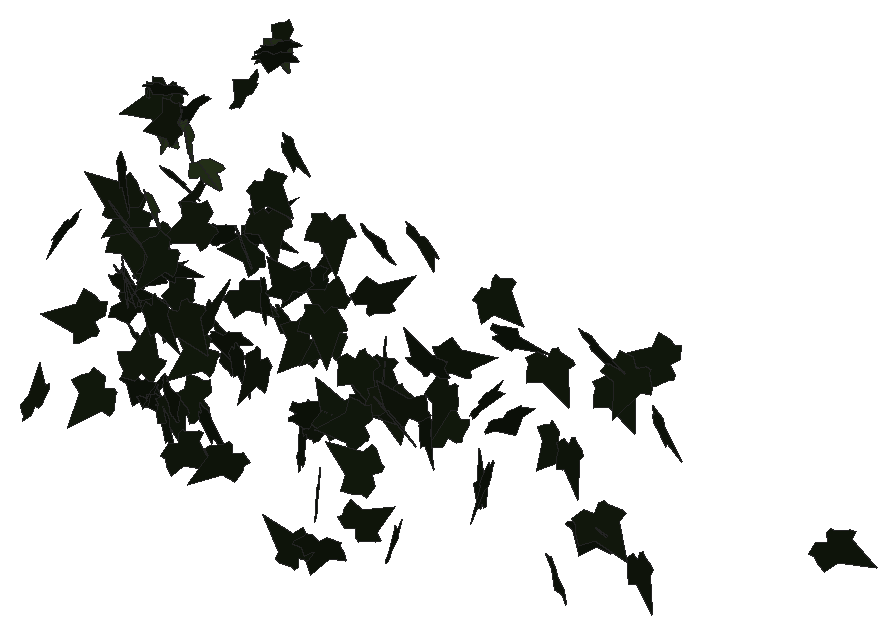
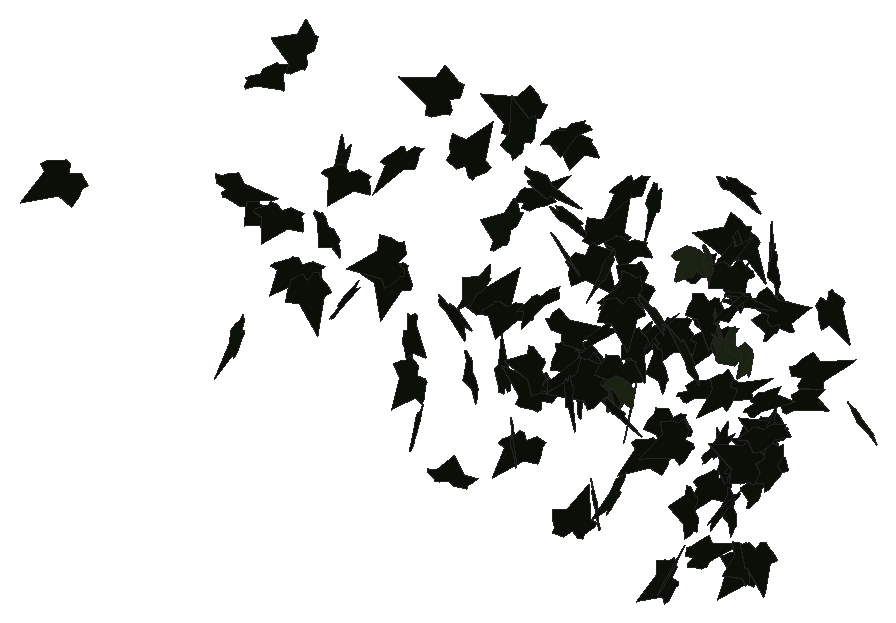
# SketchUp Ruby script. Lengths in inches.
U = 1.inch
M = Sketchup.active_model
def pt(a) = Geom::Point3d.new(a.map { |v| v * U })
def face(e, loops, mat)
  f = e.add_face(loops[0].map { |a| pt(a) })
  loops[1..].each { |l| e.add_face(l.map { |a| pt(a) }).erase! }
  f.material = f.back_material = mat if mat
  f
end
# faces: each face lists its corners as indices into pts; further lists are holes
def faces(e, pts, list, mat = nil) = list.each { |f| face(e, (f[0].is_a?(Array) ? f : [f]).map { |l| l.map { |i| pts[i] } }, mat) }
# xy, xz, yz: faces in a plane at the given z, y or x. An outline is a flat list of corners, or four numbers for a rectangle; further outlines are holes
def ring(l) = l.size == 4 ? [[l[0], l[1]], [l[2], l[1]], [l[2], l[3]], [l[0], l[3]]] : l.each_slice(2).to_a
def flat(e, list, mat, &to3) = list.each { |f| face(e, (f[0].is_a?(Array) ? f : [f]).map { |l| ring(l).map { |u, v| to3.(u, v) } }, mat) }
def xy(e, z, list, mat = nil) = flat(e, list, mat) { |x, y| [x, y, z] }
def xz(e, y, list, mat = nil) = flat(e, list, mat) { |x, z| [x, y, z] }
def yz(e, x, list, mat = nil) = flat(e, list, mat) { |y, z| [x, y, z] }
def lines(e, pts, list) = list.each { |a, b| e.add_line(pt(pts[a]), pt(pts[b])) }
# prism: a flat outline (further loops are holes) pulled along v
def prism(e, loops, v, mat = nil)
  f = face(e, loops, mat); d = Geom::Vector3d.new(v.map { |x| x * U })
  f.pushpull(f.normal.samedirection?(d) ? d.length : -d.length)
end
def box(e, o, s, mat = nil) = prism(e, [[o, [o[0] + s[0], o[1], o[2]], [o[0] + s[0], o[1] + s[1], o[2]], [o[0], o[1] + s[1], o[2]]]], [0, 0, s[2]], mat)
def at(x, y, z, deg = 0) = Geom::Transformation.translation(pt([x, y, z])) * Geom::Transformation.rotation(ORIGIN, Z_AXIS, deg.degrees)
def axes(o, x, y, z) = Geom::Transformation.new([*x, 0, *y, 0, *z, 0, *pt(o).to_a, 1])
def part(name) = M.definitions.add(name)
# library, detail: a bought-in or finely detailed component or shape, given as its bounding box
def library(name, o, s) = part(name).tap { |d| box(d.entities, o, s) }
def detail(e, o, s) = box(e.add_group.entities, o, s)
def put(e, d, t, mat = nil) = e.add_instance(d, t).tap { |i| i.material = mat if mat }
def group(e, t, mat = nil) = e.add_group.tap { |g| g.transformation = t; g.material = mat if mat }.entities
root = M.entities
M.materials.add("efeu1").color = [18, 25, 13]
M.materials.add("efeu2").color = [43, 57, 29]
c1 = part("ivyleaf_9")
p = [[1.54,2.16,1.25],[1.36,2.04,1.19],[-0.21,0.99,0.68],[-0.71,1.11,0.82],[-0.85,0.86,0.67],[-0.8,0.17,0.21],
  [-0.9,-0.01,0.1],[-0.67,-0.16,-0.02],[-0.08,-0.08,-0.05],[-0.03,-0.6,-0.4],[0.65,-0.88,-0.66],[0.83,-0.6,-0.49],
  [1.29,-0.42,-0.43],[1.8125,-0.07,-0.26],[1.21,0.44,0.15]]
faces(c1.entities,p,[[0,1,2,3,4,5,6,7,8,9,10,11,12,13,14]],"efeu1")
c2 = part("ivyleaf_10")
p = [[0,0.5,-0.03],[-0.0625,2.02,-0.43],[-0.19,2.01,-0.46],[-0.54,1.05,-0.29],[-0.52,0.625,-0.18],[-0.83,0.76,-0.28],
  [-1.16,0.64,-0.33],[-1.15,0.33,-0.24],[-0.77,-0.39,0.02],[-0.3,-0.51,0.16],[0.04,-0.48,0.23],[-0.02,2.01,-0.4375],
  [-0.06,2.01,-0.43],[0.04,-0.49,0.23],[0.67,-0.49,0.14],[1.38,0.36,-0.2],[1.375,0.51,-0.24],[0.81,0.65,-0.19],
  [0.62,0.59,-0.15],[0.6,1.09,-0.28],[0.5,1.23,-0.31]]
faces(c2.entities,p,[[0,1,2,3,4,5,6,7,8,9,10],[11,12,0,13,14,15,16,17,18,19,20]],"efeu2")
put(root,c1,axes([629.57,122.1,292.07],[-0.71361,-0.84052,0.81421],[-0.5253,-0.62208,-1.10259],[1.04568,-0.8861,0.00175]))
put(root,c1,axes([629.91,140.37,299.85],[-1.23005,0.22373,0.09712],[-0.09277,0.03263,-1.25014],[-0.22557,-1.23345,-0.01545]))
put(root,c1,axes([628.84,122,289.8],[-0.35154,-1.20696,-0.64325],[0.29676,0.58102,-1.25238],[1.33509,-0.44695,0.109]))
put(root,c1,axes([628.47,121.0625,286.31],[1.21635,-0.61794,0.36407],[0.32919,-0.15581,-1.36428],[0.63721,1.26007,0.00984]))
put(root,c1,axes([630.87,123.4375,301.76],[-1.0355,-0.05838,0.68681],[-0.66838,-0.21794,-1.02623],[0.16849,-1.2233,0.15005]))
put(root,c1,axes([629.83,125.12,302.06],[0.0302,-1.23454,0.00848],[0.00022,-0.00847,-1.23491],[1.23457,0.0302,0.00002]))
put(root,c2,axes([630.18,125.09,298.99],[-0.01245,0.99855,-0.72682],[-0.09137,-0.72561,-0.99533],[-1.23168,0.04374,0.08118]))
put(root,c2,axes([629.45,125.24,297.93],[0.68687,-0.12482,-1.01492],[1.01721,-0.04157,0.69353],[-0.10453,-1.22479,0.07989]))
put(root,c1,axes([630.79,120.64,277.54],[0.62969,0.60238,-0.88819],[-0.69997,-0.55008,-0.86932],[-0.8135,0.93958,0.06049]))
put(root,c1,axes([630.78,111.37,296.12],[-0.62437,0.95631,-0.70967],[0.367,-0.60778,-1.14189],[-1.1329,-0.72393,0.02121]))
put(root,c2,axes([630.31,138.29,300.37],[-1.17005,0.09928,-0.46292],[0.46073,-0.04536,-1.17424],[-0.10899,-1.25748,0.00581]))
put(root,c1,axes([630.16,124.96,294.55],[1.21698,-0.1043,-0.08314],[-0.07304,0.11741,-1.21644],[0.11161,1.21416,0.11049]))
put(root,c1,axes([630.16,121.86,286.3],[0.54823,1.03089,-0.57968],[0.25524,0.52075,1.16748],[1.15483,-0.60449,0.01715]))
put(root,c1,axes([631.6,122.72,303.88],[0.33423,1.02024,-0.62057],[-0.66252,-0.37772,-0.97781],[-0.99351,0.5951,0.44328]))
put(root,c1,axes([630.5625,118.77,285.53],[0.0714,0.52873,-1.29242],[0.13606,1.28531,0.53334],[1.38974,-0.153,0.01419]))
put(root,c1,axes([631.45,136.85,301.32],[0.5126,1.13395,-0.20258],[-0.2832,-0.09087,-1.22523],[-1.11655,0.54364,0.21776]))
put(root,c1,axes([632,105.65,282.48],[-1.0933,0.60329,-0.55811],[-0.49299,0.26175,1.24868],[0.65757,1.19928,0.00822]))
put(root,c2,axes([631.27,124.99,300.29],[0.83224,-0.89057,0.22858],[0.23725,-0.08987,-1.21393],[0.8883,0.85837,0.11006]))
put(root,c1,axes([631.59,120.84,276.31],[0.27096,0.53541,1.09573],[0.28579,1.06331,-0.59025],[-1.18558,0.37868,0.10814]))
put(root,c1,axes([630.96,119.13,287.47],[0.28732,-0.78886,0.90976],[0.31923,-0.85193,-0.83953],[1.16106,0.42945,0.0057]))
put(root,c1,axes([630.61,118.55,286.83],[0.47734,-0.33274,1.16148],[1.0531,-0.49756,-0.57534],[0.59222,1.15296,0.08691]))
put(root,c1,axes([632.98,116.08,296.46],[-0.20572,0.1631,1.47402],[-1.37992,0.52409,-0.25058],[-0.54327,-1.39298,0.07831]))
put(root,c1,axes([632.29,124.83,301.41],[0.09194,1.23358,-0.1325],[-0.00712,-0.13234,-1.237],[-1.24066,0.09217,-0.00272]))
put(root,c1,axes([631.58,120.79,276.125],[1.17324,0.42953,-0.0039],[-0.00984,0.01552,-1.24927],[-0.42943,1.17315,0.01795]))
put(root,c2,axes([631.95,120.25,294.83],[-0.98739,0.68872,-0.31477],[0.2713,-0.16117,-1.20365],[-0.70698,-1.02374,-0.02227]))
put(root,c1,axes([631.375,119.42,282.46],[0.68949,-0.85409,0.56382],[0.34676,-0.44466,-1.09764],[0.96287,0.77173,-0.00845]))
put(root,c1,axes([633.52,111.03,288.29],[-0.44671,-0.19552,1.39444],[-1.28089,-0.55116,-0.48761],[0.58481,-1.35655,-0.00286]))
put(root,c1,axes([633.49,120.41,291.02],[-0.5655,-0.94835,-0.6007],[-0.30568,-0.51711,1.10415],[-1.08017,0.64282,0.00202]))
put(root,c1,axes([633.6,128.8,277.14],[0.08869,-1.24031,0.50443],[0.08246,0.50964,1.23862],[-1.33643,-0.05086,0.1099]))
put(root,c1,axes([632.7,115.52,295.73],[0.84734,-0.83471,0.6193],[0.43527,-0.4406,-1.1894],[0.94383,0.95257,-0.00747]))
put(root,c1,axes([632.91,115.4375,300.49],[-0.2181,0.04436,-1.40532],[1.39566,-0.16546,-0.22182],[-0.17034,-1.41249,-0.01815]))
put(root,c1,axes([634.13,121.86,285.78],[-0.4084,-1.08907,0.62257],[0.27481,0.56116,1.16191],[-1.22399,0.48937,0.05314]))
put(root,c1,axes([633.21,128.48,277.66],[1.27932,-0.37984,0.13419],[0.12471,-0.05139,-1.33445],[0.38305,1.28531,-0.0137]))
put(root,c1,axes([634.27,120.67,302.41],[-0.2856,-0.4246,1.23886],[-0.54026,-1.11685,-0.50733],[1.19296,-0.60744,0.06683]))
put(root,c1,axes([633.48,126.62,289.375],[1.00255,0.41943,0.63751],[0.59,0.24153,-1.08674],[-0.48398,1.16327,-0.00422]))
put(root,c1,axes([635.09,128.61,301.73],[-0.30082,0.90709,0.7921],[-0.50986,0.64372,-0.9308],[-1.091,-0.55094,0.21659]))
put(root,c1,axes([634.94,132.46,303.65],[0.41526,1.03316,-0.55982],[-0.4819,-0.39179,-1.08052],[-1.07172,0.57648,0.26895]))
put(root,c1,axes([635.19,122.84,276.45],[-0.5495,-0.37194,1.16968],[-0.9516,-0.68032,-0.66338],[0.77522,-1.09876,0.0148]))
put(root,c1,axes([635.39,115.04,282.64],[-1.26897,0.13569,0.56556],[0.56179,-0.06543,1.27619],[0.15056,1.38776,0.00487]))
put(root,c1,axes([636.59,120.15,296.3125],[-0.61447,1.00994,0.46058],[-0.22136,0.40437,-1.18202],[-1.08771,-0.65283,-0.01964]))
put(root,c1,axes([636.41,108.66,284.12],[-0.88239,-1.01863,0.44685],[-0.30256,-0.32907,-1.34761],[1.07039,-0.93274,-0.01255]))
put(root,c2,axes([635.86,120.26,301.99],[-0.53403,0.43125,-1.04757],[0.60226,-0.87283,-0.66634],[-0.95951,-0.78788,0.1648]))
put(root,c1,axes([636.13,117.84,278.57],[0.46953,-1.24017,-0.27419],[-0.09916,0.25564,-1.32607],[1.26624,0.47988,-0.00217]))
put(root,c1,axes([636.3,116.72,277.78],[0.00348,0.00623,-1.3074],[1.30601,-0.06071,0.00318],[-0.06069,-1.306,-0.00639]))
put(root,c1,axes([637.63,124.92,286.27],[-0.00086,-0.1969,-1.27513],[0.33286,1.23193,-0.19046],[1.24656,-0.32909,0.04998]))
put(root,c1,axes([637.68,115.7,280.27],[-0.07045,0.03062,1.32356],[0.53196,-1.21308,0.05638],[1.21234,0.53406,0.05217]))
put(root,c2,axes([638.67,118.6875,300.8],[-1.07526,-0.33062,-0.59086],[0.56194,0.18279,-1.12491],[0.37769,-1.21321,-0.00847]))
put(root,c1,axes([638.55,118.97,277.82],[0.2918,0.06799,-1.39788],[1.39356,0.11773,0.29662],[0.12922,-1.42315,-0.04225]))
put(root,c1,axes([638.99,127.99,283.35],[1.04647,-0.84996,-0.22331],[-0.16794,0.14743,-1.34813],[0.86261,1.05982,0.00844]))
put(root,c1,axes([639.39,107.9,294.82],[-0.07187,0.09407,1.37404],[0.20254,-1.36023,0.10372],[1.36228,0.2072,0.05707]))
put(root,c1,axes([640.35,119.38,285.61],[0.78686,0.89633,-0.4783],[-0.34576,-0.3326,-1.19212],[-0.95531,0.85866,0.03751]))
put(root,c1,axes([640,114.08,277.9],[0.18253,-0.45456,-1.30556],[-0.18906,1.29631,-0.47778],[1.36944,0.23955,0.10806]))
put(root,c1,axes([641.04,115.98,297.67],[-0.92187,-0.63282,0.88161],[-0.75218,-0.46123,-1.1176],[0.78225,-1.18926,-0.03568]))
put(root,c1,axes([641.21,123.23,294.46],[0.41145,0.31446,-1.17085],[-1.1559,-0.27112,-0.47901],[-0.36561,1.21106,0.19678]))
put(root,c1,axes([641.38,115.7,286.34],[-0.94175,-0.80924,0.59251],[-0.43099,-0.40738,-1.24142],[0.90564,-1.03538,0.02535]))
put(root,c1,axes([641.52,108.63,297.0625],[-0.79287,1.04868,-0.4294],[0.26322,-0.3393,-1.31467],[-1.10219,-0.8354,-0.00508]))
put(root,c1,axes([640.79,113.07,290.61],[0.11218,-0.93482,-1.10907],[0.04056,1.11397,-0.93485],[1.44993,0.04116,0.11196]))
put(root,c1,axes([641.68,121.6,293.17],[0.27231,-1.09893,-0.7821],[0.20588,-0.75467,1.13207],[-1.33302,-0.34104,0.01508]))
put(root,c1,axes([641.88,122.3,288.79],[0.60146,-0.31189,-1.17913],[-1.07507,0.48537,-0.67677],[0.57606,1.23147,-0.03189]))
put(root,c1,axes([641.375,115.55,288.62],[-0.57207,1.30133,0.53014],[0.18601,-0.49722,1.42125],[1.39281,0.6009,0.02794]))
put(root,c1,axes([642.11,108.13,293.72],[0.89936,-1.00736,-0.6554],[-0.38415,0.53469,-1.34897],[1.13876,0.97596,0.06256]))
put(root,c1,axes([641.52,109.49,296.9375],[0.79828,-0.19444,1.12405],[1.08516,-0.29358,-0.82145],[0.35173,1.34705,-0.01678]))
put(root,c1,axes([642.53,124.6,301.5],[0.96927,-0.4397,-0.7493],[-0.60537,0.46339,-1.05502],[0.62315,1.13411,0.14057]))
put(root,c1,axes([643.63,128.48,291.51],[0.29054,-0.04804,-1.27083],[-1.26383,0.1342,-0.29402],[0.14156,1.29669,-0.01665]))
put(root,c1,axes([643.18,120.56,296.34],[0.41006,0.37396,1.25976],[0.66312,1.08044,-0.53658],[-1.13451,0.76668,0.1417]))
put(root,c1,axes([644.45,106.86,300.34],[-1.36554,-0.27359,-0.15204],[0.14957,0.02743,-1.39267],[0.27495,-1.3737,0.00248]))
put(root,c1,axes([643.91,118.78,296.59],[1.25398,0.36144,0.45038],[0.43162,0.12872,-1.30503],[-0.38366,1.32618,0.00392]))
put(root,c1,axes([644.79,115.24,287.36],[-0.19035,0.0059,-1.33006],[1.32801,0.07558,-0.18972],[0.07399,-1.34148,-0.01654]))
put(root,c1,axes([645.87,125.1,276.25],[0.71641,0.40979,1.01249],[-0.97402,-0.3083,0.81397],[0.49432,-1.20138,0.13648]))
put(root,c1,axes([646.84,121.02,275.95],[0.08276,-0.05246,1.38006],[-0.26342,1.35655,0.06737],[-1.3557,-0.26678,0.07116]))
put(root,c1,axes([645.98,118,299.18],[-0.6343,-0.83386,-0.81317],[0.5713,0.58415,-1.04465],[1.01498,-0.84991,0.07982]))
put(root,c1,axes([647.13,116.02,303.4],[0.33345,-0.77229,-1.07963],[-0.24178,1.05921,-0.83236],[1.30521,0.39352,0.12164]))
put(root,c1,axes([647.83,112.03,300.3],[0.92523,-0.20574,-0.94708],[-0.92365,0.20937,-0.94783],[0.29353,1.30735,0.00275]))
put(root,c1,axes([647.63,114.7,287.85],[0.13237,-0.12922,-1.4706],[0.94366,-1.12806,0.18406],[-1.13528,-0.95272,-0.01848]))
put(root,c1,axes([650.03,121.16,290.95],[-0.14893,0.16182,1.37776],[-1.26331,0.55665,-0.20194],[-0.57311,-1.26908,0.0871]))
put(root,c1,axes([649.73,118.18,289.09],[-0.53998,-1.0524,0.877],[-0.25218,-0.8502,-1.17551],[1.3465,-0.58126,0.13154]))
put(root,c1,axes([650.6,117.37,295.99],[0.05131,0.73717,-1.19645],[-0.06889,-1.19449,-0.73891],[-1.40363,0.08557,-0.00747]))
put(root,c1,axes([650.02,126.01,283.1],[-0.03203,-0.54579,-1.27663],[0.08569,1.27376,-0.54671],[1.38576,-0.09138,0.0043]))
put(root,c1,axes([651.04,126.14,282.5625],[-0.03493,0.08559,1.33642],[-0.11956,1.33134,-0.08839],[-1.33381,-0.12158,-0.02708]))
put(root,c1,axes([651.18,106.51,284.18],[-0.13,0.2299,-1.40122],[-0.18909,-1.39735,-0.21172],[-1.40731,0.16652,0.15789]))
put(root,c1,axes([651.28,114.3125,295.99],[0.54137,0.33338,1.21324],[-1.16094,-0.37685,0.62159],[0.48508,-1.27398,0.13362]))
put(root,c1,axes([651.92,118.83,296.89],[-1.0708,0.40282,-0.79971],[-0.75211,0.27192,1.14403],[0.48593,1.30851,0.00845]))
put(root,c1,axes([650.78,115.84,283.7],[1.01894,0.27131,0.93726],[0.91068,0.22214,-1.05434],[-0.35034,1.36651,-0.0147]))
put(root,c1,axes([653.55,117.6,283.22],[-0.7675,-1.13058,0.27093],[0.17076,0.21149,1.3663],[-1.14998,0.78596,0.02206]))
put(root,c1,axes([654.02,127.27,295.93],[0.36075,-1.11878,0.81087],[0.53975,-0.65736,-1.14711],[1.27194,0.59626,0.2568]))
put(root,c1,axes([654.13,119.07,285.17],[0.49177,-0.09644,-1.30697],[1.2277,0.5223,0.4234],[0.45851,-1.29507,0.26808]))
put(root,c1,axes([655.11,112.73,278.68],[-0.00944,0.42488,1.40918],[0.03048,-1.40885,0.42499],[1.47153,0.03191,0.00024]))
put(root,c1,axes([656.24,127.9375,278.34],[-1.28968,-0.24558,0.32847],[0.32211,0.06434,1.31286],[-0.25386,1.3293,-0.00287]))
put(root,c1,axes([655.93,113.54,303.95],[-0.20806,-1.37478,-0.41183],[0.09839,0.40149,-1.38998],[1.43176,-0.22737,0.03568]))
put(root,c1,axes([656.01,116.56,290.04],[0.22019,-1.24411,-0.66524],[-0.02716,0.66943,-1.26094],[1.41054,0.2071,0.07957]))
put(root,c1,axes([657.875,106.68,277.28],[0.09719,-0.04628,1.45505],[-1.23228,0.77382,0.10692],[-0.77511,-1.23604,0.01246]))
put(root,c1,axes([657.59,111.99,295.25],[-1.44348,0.02843,0.02136],[-0.0214,-0.00196,-1.44376],[-0.0284,-1.44364,0.00238]))
put(root,c1,axes([659.26,116.79,288.07],[-0.45373,-1.04339,-0.84297],[0.37834,0.75421,-1.13717],[1.28691,-0.58961,0.03711]))
put(root,c1,axes([660.17,106.64,279.3125],[0.728,0.85294,-0.96205],[-0.62846,-0.72842,-1.12137],[-1.12164,0.96173,0.0039]))
put(root,c1,axes([658.99,115.03,302.71],[1.28246,-0.27246,-0.62526],[0.63183,-0.02687,1.30765],[-0.25685,-1.42651,0.09479]))
put(root,c1,axes([659.82,107.73,299.43],[-0.91788,-0.68179,-0.92156],[0.71199,0.58619,-1.14283],[0.89843,-1.1611,-0.03584]))
put(root,c1,axes([659.37,112.46,277.81],[-0.18462,0.07935,1.36237],[1.32698,-0.3105,0.19791],[0.31858,1.33931,-0.03484]))
put(root,c1,axes([659.54,120.87,283.86],[-0.22321,-0.10583,-1.41746],[1.41954,-0.09002,-0.21682],[-0.07273,-1.4321,0.11838]))
put(root,c1,axes([661.42,116.36,287],[0.71947,0.01913,1.28158],[-1.2811,-0.03512,0.71972],[0.03998,-1.4693,-0.00052]))
put(root,c1,axes([661.9,125.08,284.46],[0.29295,1.03713,0.86974],[0.25105,0.8328,-1.07765],[-1.33006,0.38562,-0.01184]))
put(root,c1,axes([662.56,119.93,288.35],[-1.24159,-0.11695,-0.761],[0.75735,0.07449,-1.24708],[0.13864,-1.45434,-0.00268]))
put(root,c1,axes([663.79,122.86,277.48],[-0.01809,-0.69878,1.18156],[0.09215,1.17838,0.69831],[-1.36963,0.08851,0.03138]))
put(root,c1,axes([663.41,111.875,277.6],[0.11241,0.72856,1.12827],[-0.13382,-1.12051,0.73688],[1.33637,-0.17349,-0.02112]))
put(root,c1,axes([662.98,109.57,300.94],[0.08299,-0.10046,1.48711],[1.44472,0.3717,-0.05551],[-0.36655,1.44229,0.11789]))
put(root,c1,axes([665.55,105.31,292.39],[-1.18956,0.33144,0.84646],[-0.81045,0.24472,-1.23478],[-0.41172,-1.43933,-0.01503]))
put(root,c1,axes([664.04,110.61,290.81],[0.74753,-0.95085,0.86477],[0.67089,-0.56463,-1.20077],[1.09629,0.99389,0.14516]))
put(root,c1,axes([665.51,123.17,292.83],[1.13054,-0.07307,0.83744],[0.83769,-0.01914,-1.13255],[0.07012,1.40679,0.02809]))
put(root,c1,axes([667.47,103.92,289.34],[-0.73983,-1.24347,-0.37199],[-0.13584,-0.35165,1.44562],[-1.29079,0.74971,0.06108]))
put(root,c1,axes([667.8,111.26,295.8],[0.89307,-0.46326,1.08855],[-0.97781,0.47866,1.00593],[-0.6659,-1.32416,-0.0172]))
put(root,c1,axes([668.12,118.22,283.51],[-0.61256,0.43554,-1.27982],[1.03818,-0.74842,-0.75161],[-0.86592,-1.20542,0.00424]))
put(root,c1,axes([668.18,118.68,299.82],[0.34401,-0.78362,-1.19815],[-0.2587,1.17795,-0.84468],[1.40808,0.40787,0.13753]))
put(root,c1,axes([669.57,118.48,288.76],[0.44627,1.40732,0.05684],[0.01659,0.05436,-1.47638],[-1.40837,0.44658,0.00062]))
put(root,c1,axes([672.22,121.94,285.9375],[-0.23191,-0.93222,1.02547],[-0.14324,-1.01804,-0.95786],[1.37845,-0.26262,0.07299]))
put(root,c1,axes([671.9,108.57,299.14],[0.44057,-0.06293,1.39339],[1.37865,-0.20217,-0.44504],[0.21173,1.44733,-0.00158]))
put(root,c1,axes([674.14,118.35,295.76],[-0.4721,-0.72282,-1.14476],[0.61493,0.96561,-0.8633],[1.20616,-0.77522,-0.00794]))
put(root,c1,axes([675.87,130.14,285.72],[1.21281,-0.60857,-0.66557],[-0.59992,0.28841,-1.35689],[0.67337,1.35303,-0.01013]))
put(root,c1,axes([677.2,117.2,289.27],[-0.59447,-0.21062,-1.29138],[1.27994,0.20086,-0.62196],[0.27164,-1.40738,0.10449]))
put(root,c1,axes([677.67,122.58,292.9],[-0.48071,-0.78955,-1.10573],[0.57989,0.94147,-0.92437],[1.22872,-0.75322,0.00366]))
put(root,c1,axes([679.75,116.49,283.02],[0.72924,0.61538,-1.08606],[-0.94092,-0.55557,-0.94658],[-0.82029,1.18433,0.12027]))
put(root,c1,axes([681.08,124.99,294.88],[-0.82753,0.11429,1.17983],[-1.1635,0.19668,-0.83513],[-0.22654,-1.42762,-0.02061]))
put(root,c1,axes([680.38,116.67,284.45],[-0.03693,-0.92342,-1.19789],[0.47004,1.13191,-0.88705],[1.43761,-0.39381,0.25925]))
put(root,c1,axes([682.29,113.79,301.91],[0.77386,-0.70973,1.07232],[0.85024,-0.65651,-1.04811],[0.96472,1.14792,0.06356]))
put(root,c1,axes([685.08,115.66,299.83],[-0.73122,-1.31011,0.1541],[-0.07104,-0.13683,-1.50035],[1.31723,-0.73465,0.00463]))
put(root,c1,axes([685.82,104.99,285.75],[-0.05594,-0.49184,1.39855],[0.3286,-1.36885,-0.46825],[1.44564,0.29211,0.16055]))
put(root,c1,axes([688.5,111.93,285.09],[-0.54133,-0.09997,-1.35765],[1.32489,0.29708,-0.55014],[0.31285,-1.43108,-0.01936]))
put(root,c1,axes([700.9,120.77,287.34],[0.00805,-0.02791,-1.51187],[0.41027,1.45522,-0.02468],[1.4554,-0.41007,0.01532]))
